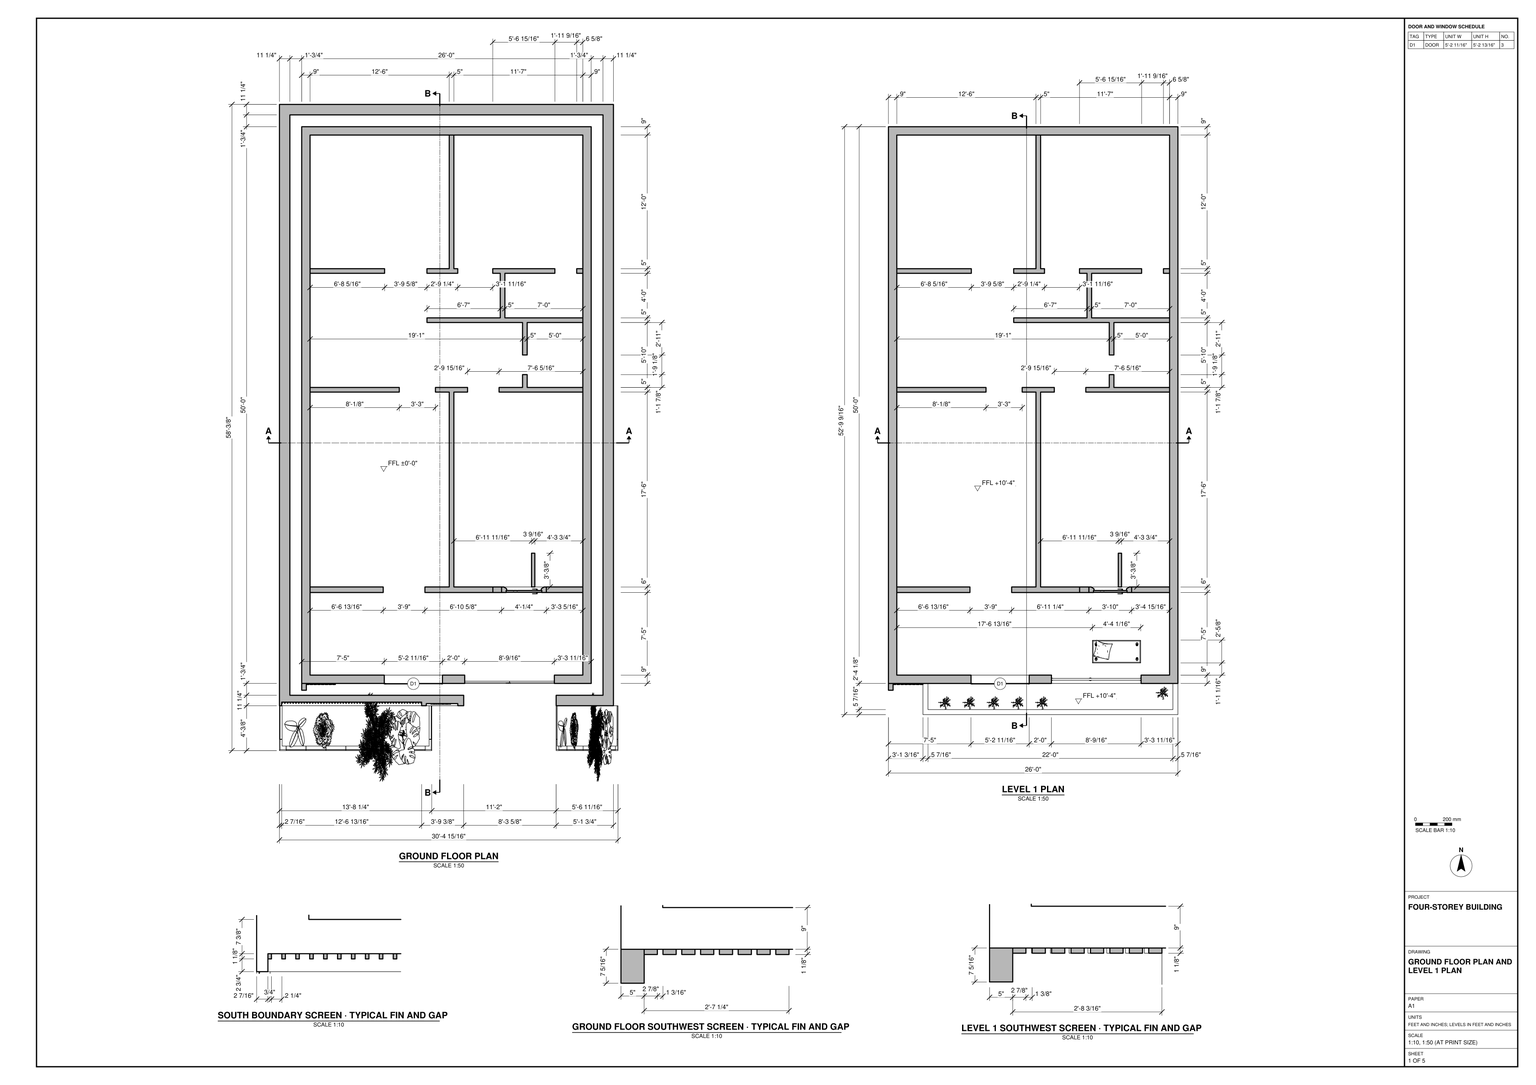
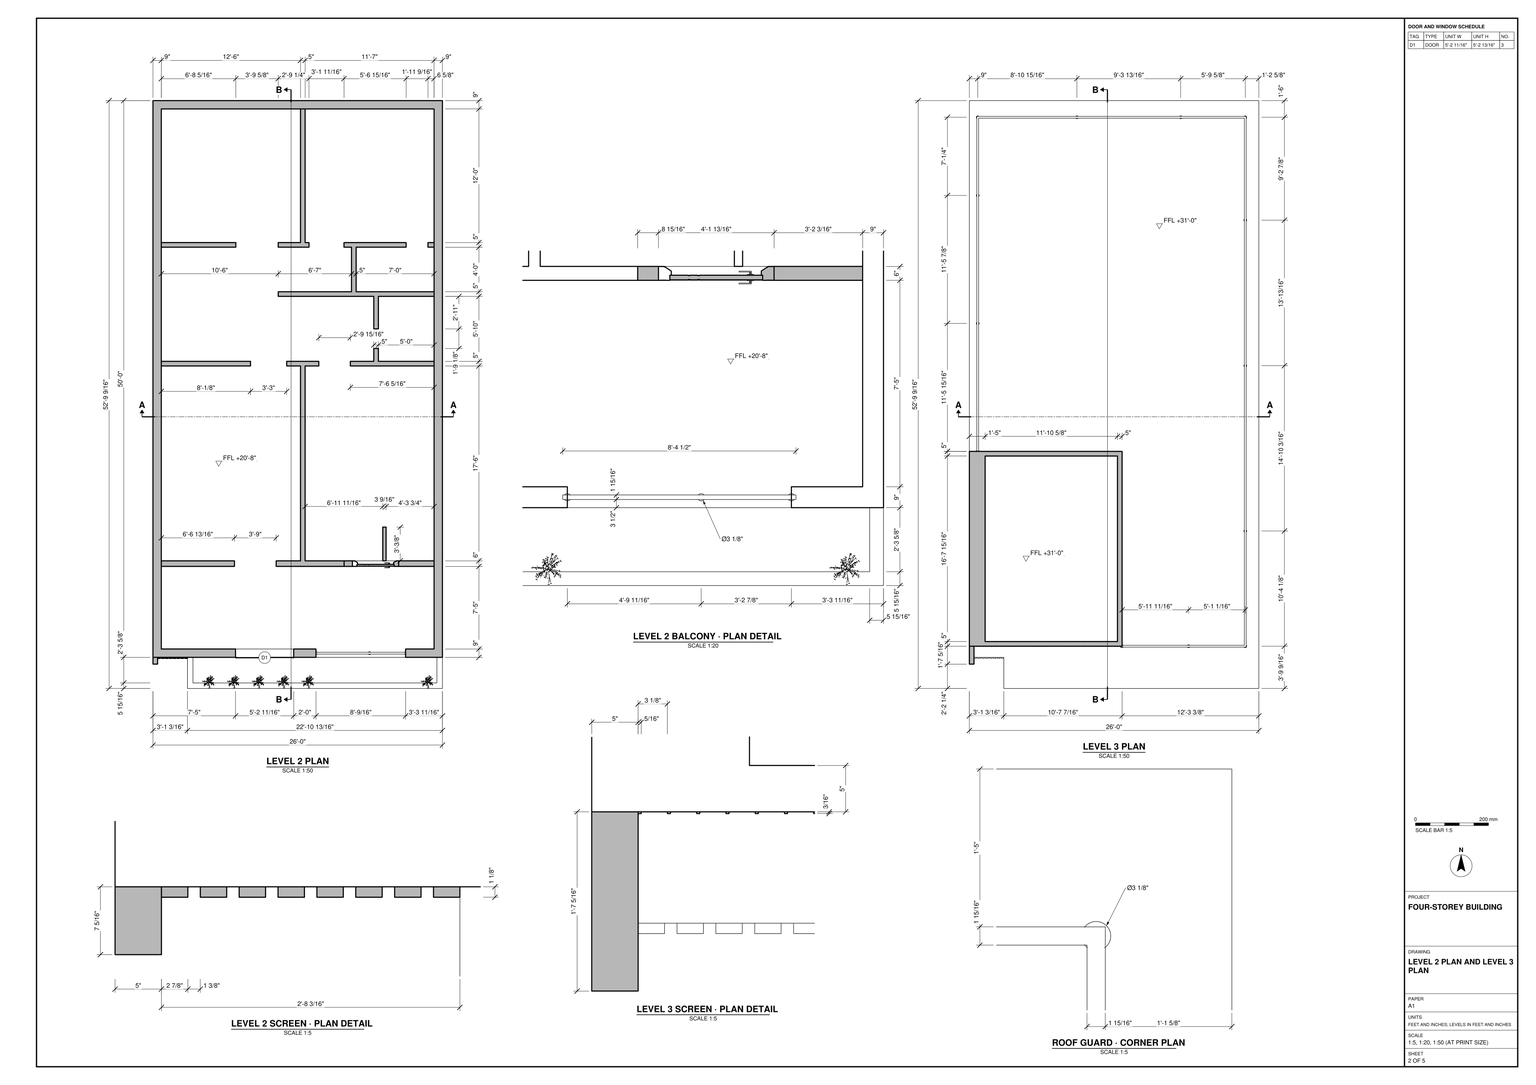
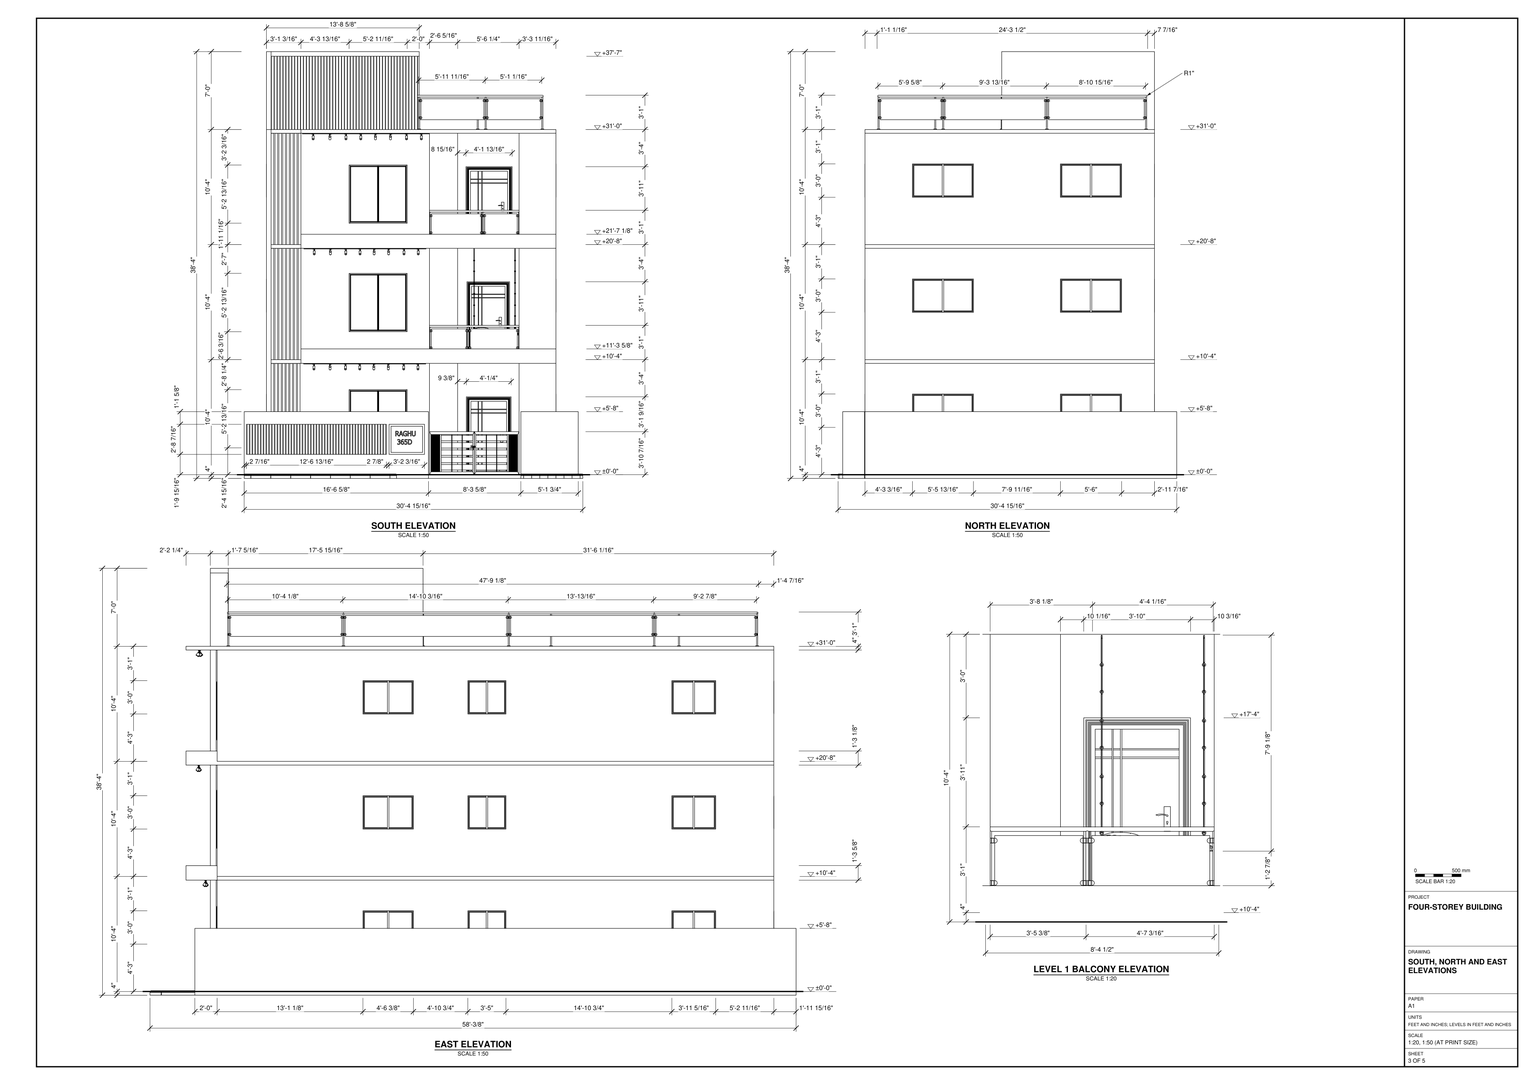
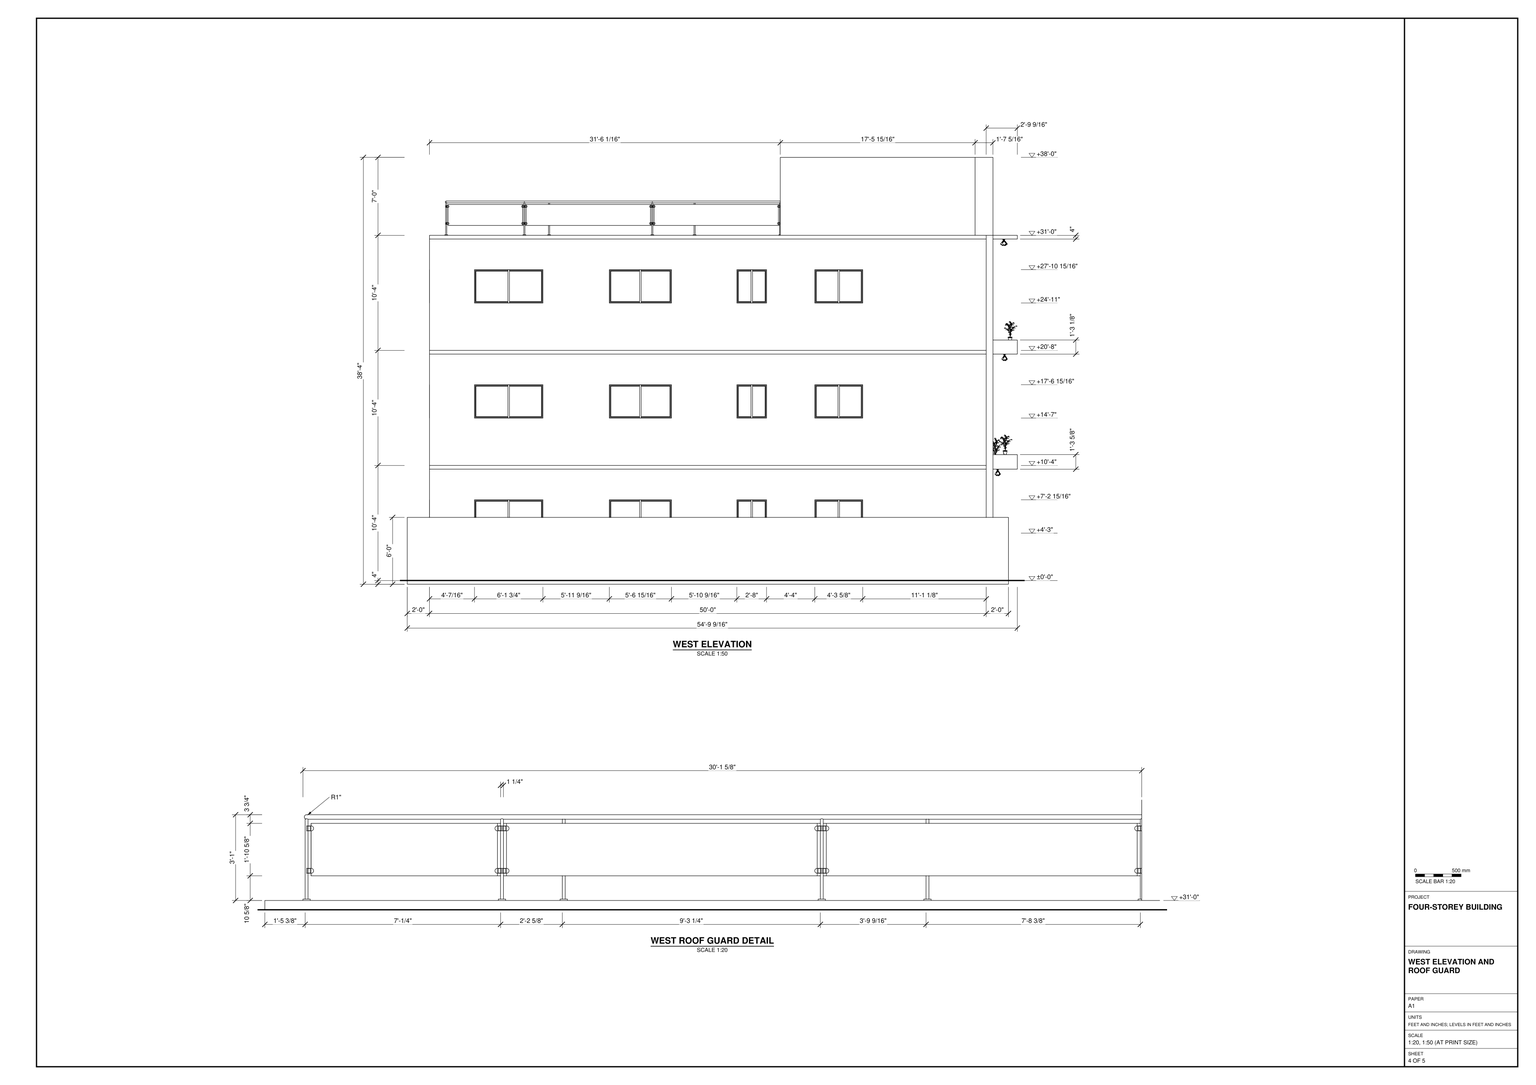
Build the four-storey building in SketchUp from task_files/diagram_01.pdf. Work in feet and inches, with the south entrance frontage along X and the building depth along Y. The overall model, including the boundary and frontage elements, is 30'-4 15/16" wide, 60'-9 5/8" deep and 38'-4" high. Set the finished floor levels to ±0'-0", +10'-4", +20'-8" and +31'-0".

Use the plans to set out the three lower floors. Model the perimeter walls, internal partitions and floor slabs at the thicknesses drawn. Preserve the passage openings between rooms, and use the elevations to place the exterior doors and windows. Model the projecting south balcony slabs, their guards and the narrow band of vertical fins at the southwest corner. At the top level, distinguish the screened southwest enclosure from the open roof terrace and follow the roof guard detail around the exposed edges.

Include the boundary walls, south entrance gate, finned boundary screen and planting beds in their plan positions. Place the swing shown near the southeast corner of the Level 1 front room. Model circulation, built-in joinery and main furniture where indicated on the sheets. Decor and loose items, including plants and lights, may be represented by any suitable library components.

Keep shell elements such as walls, slabs and roof separate as groups or components, and group each furniture or joinery piece separately. Use components for repeated parts such as screen fins and window units. Save one SketchUp model as output_files/four_storey_building_south_balconies_and_roof_terrace.skp.

# SketchUp Ruby script. Lengths in inches.
U = 1.inch
M = Sketchup.active_model
def pt(a) = Geom::Point3d.new(a.map { |v| v * U })
def face(e, loops, mat)
  f = e.add_face(loops[0].map { |a| pt(a) })
  loops[1..].each { |l| e.add_face(l.map { |a| pt(a) }).erase! }
  f.material = f.back_material = mat if mat
  f
end
# faces: each face lists its corners as indices into pts; further lists are holes
def faces(e, pts, list, mat = nil) = list.each { |f| face(e, (f[0].is_a?(Array) ? f : [f]).map { |l| l.map { |i| pts[i] } }, mat) }
# xy, xz, yz: faces in a plane at the given z, y or x. An outline is a flat list of corners, or four numbers for a rectangle; further outlines are holes
def ring(l) = l.size == 4 ? [[l[0], l[1]], [l[2], l[1]], [l[2], l[3]], [l[0], l[3]]] : l.each_slice(2).to_a
def flat(e, list, mat, &to3) = list.each { |f| face(e, (f[0].is_a?(Array) ? f : [f]).map { |l| ring(l).map { |u, v| to3.(u, v) } }, mat) }
def xy(e, z, list, mat = nil) = flat(e, list, mat) { |x, y| [x, y, z] }
def xz(e, y, list, mat = nil) = flat(e, list, mat) { |x, z| [x, y, z] }
def yz(e, x, list, mat = nil) = flat(e, list, mat) { |y, z| [x, y, z] }
def lines(e, pts, list) = list.each { |a, b| e.add_line(pt(pts[a]), pt(pts[b])) }
# prism: a flat outline (further loops are holes) pulled along v
def prism(e, loops, v, mat = nil)
  f = face(e, loops, mat); d = Geom::Vector3d.new(v.map { |x| x * U })
  f.pushpull(f.normal.samedirection?(d) ? d.length : -d.length)
end
def box(e, o, s, mat = nil) = prism(e, [[o, [o[0] + s[0], o[1], o[2]], [o[0] + s[0], o[1] + s[1], o[2]], [o[0], o[1] + s[1], o[2]]]], [0, 0, s[2]], mat)
def at(x, y, z, deg = 0) = Geom::Transformation.translation(pt([x, y, z])) * Geom::Transformation.rotation(ORIGIN, Z_AXIS, deg.degrees)
def axes(o, x, y, z) = Geom::Transformation.new([*x, 0, *y, 0, *z, 0, *pt(o).to_a, 1])
def part(name) = M.definitions.add(name)
# library, detail: a bought-in or finely detailed component or shape, given as its bounding box
def library(name, o, s) = part(name).tap { |d| box(d.entities, o, s) }
def detail(e, o, s) = box(e.add_group.entities, o, s)
def put(e, d, t, mat = nil) = e.add_instance(d, t).tap { |i| i.material = mat if mat }
def group(e, t, mat = nil) = e.add_group.tap { |g| g.transformation = t; g.material = mat if mat }.entities
root = M.entities
M.materials.add("PDM_Concrete_02N").color = [160, 160, 159]
M.materials.add("PDM_Concrete_02N-1").color = [160, 160, 159]
M.materials.add("PDM_Grass_03").color = [113, 137, 58]
M.materials.add("[0022_Maroon]").color = [128, 0, 0]
M.materials.add("[0041_Chocolate]").color = [210, 105, 30]
M.materials.add("[0132_LightGray]").color = [169, 169, 169]
M.materials.add("[0135_DarkGray]").color = [81, 81, 81]
M.materials.add("[0136_Charcoal]").color = [35, 35, 35]
M.materials.add("[Marble Carrara Floor Tile]").color = [204, 208, 219]
M.materials.add("[Mirror 02]").color = [229, 229, 229]
M.materials.add("[Terrazzo Light Blue]").color = [196, 214, 227]
M.materials.add("[Translucent Glass Tinted]").color = [8, 201, 241]
M.materials["[Translucent Glass Tinted]"].alpha = 0.48
M.materials.add("[Wood Cherry Original]").color = [152, 86, 42]
c1 = part("PENTEK_RP Fineline 50S_Sliding_DoorCase_E1")
box(c1.entities,[0,0,0],[1.51,3.66,99.27],"[0135_DarkGray]")
c2 = part("PENTEK_RP Fineline 50S_SlidingDooe_Case_E2")
box(c2.entities,[0,0,0],[96.25,3.66,1.51],"[0135_DarkGray]")
c3 = part("pentek_RP Fineline 50S_SlidingDoor_Case")
put(c3.entities,c1,at(97.76,0,0))
put(c3.entities,c2,at(1.51,0,0))
put(c3.entities,c1,at(0,0,0))
put(c3.entities,c2,at(1.51,0,97.76))
c4 = part("PENTEK_RP Fineline 50S_SlidingDoor_GlazingBead_2")
box(c4.entities,[0,0,0],[0.56,0.59,94.39],"[0135_DarkGray]")
c5 = part("PENTEK_RP Fineline 50S_SlidingDoor_Glass")
box(c5.entities,[0,0,0],[46.58,0.16,94.39],"[Translucent Glass Tinted]")
c6 = part("PENTEK_RP Fineline 50S_SlidingDoor_GlazingBead")
box(c6.entities,[0,0,0],[45.47,0.59,0.56],"[0135_DarkGray]")
c7 = part("PENTEK_RP Fineline 50S_SlidingDoor_Leaf_E1")
xy(c7.entities,0,[[0,0,0.93,1.97],[0.93,1.57,1.49,1.97]],"[0135_DarkGray]")
xy(c7.entities,96.25,[[0,0,0.93,0,0.93,1.57,1.49,1.57,1.49,1.97,0,1.97]],"[0135_DarkGray]")
xz(c7.entities,0,[[0,0,0.93,96.25]],"[0135_DarkGray]")
xz(c7.entities,1.57,[[0.93,0,1.49,95.32],[0.93,95.32,1.49,96.25]],"[0135_DarkGray]")
xz(c7.entities,1.97,[[0,0,1.49,96.25]],"[0135_DarkGray]")
yz(c7.entities,0,[[0,0,1.97,96.25]],"[0135_DarkGray]")
yz(c7.entities,0.93,[[0,0,1.57,0.93],[0,0.93,1.57,95.32],[0,95.32,1.57,96.25]],"[0135_DarkGray]")
yz(c7.entities,1.49,[[1.57,0,1.97,95.32],[1.57,95.32,1.97,96.25]],"[0135_DarkGray]")
c8 = part("PENTEK_RP Fineline 50S_SlidingDoor_Leaf_E2")
xy(c8.entities,0,[[0,0,0,1.57,0.56,1.57,0.56,1.97,46.02,1.97,46.02,1.57,46.58,1.57,46.58,0]],"[0135_DarkGray]")
xy(c8.entities,0.93,[[0,0,46.58,1.57]],"[0135_DarkGray]")
xy(c8.entities,1.49,[[0.56,1.57,46.02,1.97]],"[0135_DarkGray]")
xz(c8.entities,0,[[0,0,46.58,0.93]],"[0135_DarkGray]")
xz(c8.entities,1.57,[[0,0,0.56,0.93],[46.02,0,46.58,0.93],[0.56,0.93,46.02,1.49]],"[0135_DarkGray]")
xz(c8.entities,1.97,[[0.56,0,46.02,1.49]],"[0135_DarkGray]")
yz(c8.entities,0,[[0,0,1.57,0.93]],"[0135_DarkGray]")
yz(c8.entities,0.56,[[1.57,0,1.97,0.93],[1.57,0.93,1.97,1.49]],"[0135_DarkGray]")
yz(c8.entities,46.02,[[1.57,0,1.97,0.93],[1.57,0.93,1.97,1.49]],"[0135_DarkGray]")
yz(c8.entities,46.58,[[0,0,1.57,0.93]],"[0135_DarkGray]")
c9 = part("PENTEK_RP Fineline S_SlidingDoor_Leaf1")
put(c9.entities,c4,at(0.93,0,0.93))
put(c9.entities,c4,at(46.96,0,0.93))
put(c9.entities,c5,at(1.49,1.42,0.93))
put(c9.entities,c6,at(1.49,0,0.93))
put(c9.entities,c5,at(1.49,0.59,0.93),"[Terrazzo Light Blue]")
put(c9.entities,c7,at(0,0,0))
put(c9.entities,c7,axes([48.44,0,0],[-1,0,0],[0,1,0],[0,0,1]))
put(c9.entities,c8,axes([0.93,0,96.25],[1,0,0],[0,1,0],[0,0,-1]))
put(c9.entities,c8,at(0.93,0,0))
put(c9.entities,c6,at(1.49,0,94.77))
c10 = part("PENTEK_RP Fineline 50S_SlidingDoor_Leaf2")
put(c10.entities,c5,at(1.49,1.42,0.93))
put(c10.entities,c6,at(1.49,0,94.77))
put(c10.entities,c4,at(46.96,0,0.93))
put(c10.entities,c5,at(1.49,0.59,0.93),"[Mirror 02]")
put(c10.entities,c4,at(0.93,0,0.93))
put(c10.entities,c7,at(0,0,0))
put(c10.entities,c7,axes([48.44,0,0],[-1,0,0],[0,1,0],[0,0,1]))
put(c10.entities,c6,at(1.49,0,0.93))
put(c10.entities,c8,axes([0.93,0,96.25],[1,0,0],[0,1,0],[0,0,-1]))
put(c10.entities,c8,at(0.93,0,0))
c11 = part("PENTEK - Slimmest Steel Sliding Door / Window\#1")
put(c11.entities,c3,at(0,-1.88,-0.09))
put(c11.entities,c9,at(1.51,-2.27,1.42),"[0041_Chocolate]")
put(c11.entities,c10,at(49.32,-0.3,1.42),"[0041_Chocolate]")
c12 = library("track spot lights",[-0.02,-0.08,0],[184.83,7.92,7.16])
c13 = part("Group136\#1")
p = [[0,0,0],[0,0,-16.31],[-4.35,0,-16.31],[28.32,-24.48,0],[-28.32,-24.48,0],[28.32,24.48,0],
  [28.32,0,0],[-28.32,24.48,0],[4.35,0,-16.31],[-28.32,0,0],[0,0,-26.4]]
lines(c13.entities,p,[[0,1],[1,2],[3,4],[5,6],[7,5],[1,8],[9,0],[0,6],[8,10],[4,9],[6,3],[2,10],
  [9,7]])
c14 = part("Rectangle Light")
put(c14.entities,c13,at(0,0,0))
c15 = part("Group138\#1")
p = [[0,0,0],[0,0,-9.13],[-1.42,0,-9.13],[9.23,-20.33,0],[-9.23,-20.33,0],[9.23,20.33,0],
  [9.23,0,0],[-9.23,20.33,0],[1.42,0,-9.13],[-9.23,0,0],[0,0,-14.78]]
lines(c15.entities,p,[[0,1],[1,2],[3,4],[5,6],[7,5],[1,8],[9,0],[0,6],[8,10],[4,9],[6,3],[2,10],
  [9,7]])
c16 = part("Rectangle Light\#1")
put(c16.entities,c15,at(0,0,0))
c17 = part("Group140\#1")
p = [[0,0,0],[0,0,-16.18],[-6.125,0,-16.18],[39.875,-12.51,0],[-39.875,-12.51,0],[39.875,12.51,0],
  [39.875,0,0],[-39.875,12.51,0],[6.125,0,-16.18],[-39.875,0,0],[0,0,-26.19]]
lines(c17.entities,p,[[0,1],[1,2],[3,4],[5,6],[7,5],[1,8],[9,0],[0,6],[8,10],[4,9],[6,3],[2,10],
  [9,7]])
c18 = part("Rectangle Light\#2")
put(c18.entities,c17,at(0,0,0))
c19 = part("Group142\#1")
p = [[0,0,0],[0,0,-9.18],[-1.75,0,-9.18],[11.4,-18.32,0],[-11.4,-18.32,0],[11.4,18.32,0],
  [11.4,0,0],[-11.4,18.32,0],[1.75,0,-9.18],[-11.4,0,0],[0,0,-14.86]]
lines(c19.entities,p,[[0,1],[1,2],[3,4],[5,6],[7,5],[1,8],[9,0],[0,6],[8,10],[4,9],[6,3],[2,10],
  [9,7]])
c20 = part("Rectangle Light\#3")
put(c20.entities,c19,at(0,0,0))
c21 = part("Group144\#1")
p = [[0,0,0],[0,0,-17.3125],[-6.92,0,-17.3125],[45.07,-10.98,0],[-45.07,-10.98,0],[45.07,10.98,0],
  [45.07,0,0],[-45.07,10.98,0],[6.92,0,-17.3125],[-45.07,0,0],[0,0,-28.02]]
lines(c21.entities,p,[[0,1],[1,2],[3,4],[5,6],[7,5],[1,8],[9,0],[0,6],[8,10],[4,9],[6,3],[2,10],
  [9,7]])
c22 = part("Rectangle Light\#4")
put(c22.entities,c21,at(0,0,0))
c23 = part("Group146\#1")
p = [[0,0,0],[0,0,-17.125],[-5.35,0,-17.125],[34.8,-20.64,0],[-34.8,-20.64,0],[34.8,20.64,0],
  [34.8,0,0],[-34.8,20.64,0],[5.35,0,-17.125],[-34.8,0,0],[0,0,-27.72]]
lines(c23.entities,p,[[0,1],[1,2],[3,4],[5,6],[7,5],[1,8],[9,0],[0,6],[8,10],[4,9],[6,3],[2,10],
  [9,7]])
c24 = part("Rectangle Light\#5")
put(c24.entities,c23,at(0,0,0))
c25 = part("255x125 HB kerb.skp\#1")
prism(c25.entities,[[[35.98,4.92,10.04],[35.98,1.15,10.04],[35.98,0.9375,9.96],[35.98,0.8125,9.77],[35.98,0,6.1],[35.98,0,0],[35.98,4.92,0]]],[-35.98,0,0])
c26 = part("305x125 HB external kerb.skp")
xy(c26.entities,0,[[0,0,0,4.92,7.09,4.92,7.09,12.01,12.01,12.01,12.01,0]])
xy(c26.entities,10.04,[[0,1.15,10.86,1.15,10.86,12.01,7.09,12.01,7.09,4.92,0,4.92]])
xz(c26.entities,0,[[0,0,12.01,6.1]])
xz(c26.entities,4.92,[[0,0,7.09,10.04]])
xz(c26.entities,12.01,[[7.09,0,7.09,10.04,10.86,10.04,11.07,9.96,11.19,9.77,12.01,6.1,12.01,0]])
yz(c26.entities,0,[[0,0,0,6.1,0.8125,9.77,0.9375,9.96,1.15,10.04,4.92,10.04,4.92,0]])
yz(c26.entities,7.09,[[4.92,0,12.01,10.04]])
yz(c26.entities,12.01,[[0,0,12.01,6.1]])
p = [[0,0.8125,9.77],[0,0,6.1],[12.01,0,6.1],[11.19,0.8125,9.77],[12.01,12.01,6.1],[11.19,12.01,9.77],
  [0,0.9375,9.96],[11.07,0.9375,9.96],[11.07,12.01,9.96],[0,1.15,10.04],[10.86,1.15,10.04],[10.86,12.01,10.04]]
faces(c26.entities,p,[[0,1,2,3],[3,2,4,5],[6,0,3,7],[7,3,5,8],[9,6,7,10],[10,7,8,11]])
c27 = library("Vase_plant.skp",[-29.68,-24.2,-1.65],[45.82,40.28,40.94])
c28 = library("Aralia.skp\#1",[-13.5,-14.26,0],[27.8,28.98,28.64])
c29 = library("bamboo2.skp\#1",[-10.58,-11.09,0],[94.17,118.22,79.29])
c30 = library("Monstera.skp\#1",[-40.08,-33.23,-2.65],[72.39,71.54,61.35])
c31 = part("flowers")
xy(c31.entities,8.27,[[6.7,5.98,275.44,49.6875]],"PDM_Grass_03")
xz(c31.entities,5.98,[[6.7,0,275.44,8.27]])
xz(c31.entities,49.6875,[[6.7,0,6.9375,8.27],[6.9375,0,275.44,8.27],[6.9375,8.27,275.44,10.04]],"PDM_Concrete_02N")
yz(c31.entities,6.7,[[5.98,0,49.6875,8.27]])
yz(c31.entities,275.44,[[5.98,0,49.6875,8.27]])
p = [[2.02,1.3,0],[2.02,40.67,0]]
lines(c31.entities,p,[[0,1]])
put(c31.entities,c25,at(14.42,1.3,0),"PDM_Concrete_02N-1")
put(c31.entities,c26,at(268.36,1.3,0),"PDM_Concrete_02N-1")
put(c31.entities,c26,at(2.02,13.31,0,-90),"PDM_Concrete_02N-1")
put(c31.entities,c25,at(50.8,1.3,0),"PDM_Concrete_02N-1")
put(c31.entities,c25,at(87.18,1.3,0),"PDM_Concrete_02N-1")
put(c31.entities,c25,at(123.55,1.3,0),"PDM_Concrete_02N-1")
put(c31.entities,c25,at(159.77,1.3,0),"PDM_Concrete_02N-1")
put(c31.entities,c25,at(195.99,1.3,0),"PDM_Concrete_02N-1")
put(c31.entities,c25,at(232.21,1.3,0),"PDM_Concrete_02N-1")
put(c31.entities,c25,at(280.36,13.7,0,90),"PDM_Concrete_02N-1")
put(c31.entities,c25,at(2.02,49.6875,0,-90),"PDM_Concrete_02N-1")
put(c31.entities,c27,at(36.73,27.57,8.27))
put(c31.entities,c28,axes([82.45,23.77,8.27],[1.4,0,0],[0,1.43,0],[0,0,1.63]))
put(c31.entities,c29,at(140.88,-31.91,8.22))
put(c31.entities,c30,at(227.05,18.7,8.27,-180))
c32 = library("TRADITIONAL SWING",[0,0,0],[52.04,24.99,103.38])
c33 = part("Group\#6")
box(c33.entities,[0,0,0],[6.61,5,120])
c34 = part("Group\#9")
box(c34.entities,[0,0,0],[3.5625,36.37,120])
c35 = part("Group\#7")
prism(c35.entities,[[[33.23,5,0],[33.23,0,0],[0,0,0],[0,5,0],[24.03,5,0],[24.03,149,0],[29.03,149,0],[29.03,5,0]]],[0,0,120])
c36 = part("Group\#8")
box(c36.entities,[0,0,0],[96.15,5,120])
c37 = library("Group\#42",[0,-1.57,0],[96.98,7.57,120])
c38 = part("Group\#3")
prism(c38.entities,[[[0,40,0],[79,40,0],[79,88,0],[70.89,88,0],[70.89,93,0],[137.86,93,0],[137.86,88,0],[84,88,0],[84,40,0],[168,40,0],[168,35,0],[108,35,0],[108,0,0],[103,0,0],[103,35,0],[0,35,0]]],[0,0,120])
c39 = part("Group\#4")
box(c39.entities,[0,0,0],[80.33,5,120])
c40 = part("Group\#5")
prism(c40.entities,[[[25.29,18.85,0],[30.29,18.85,0],[30.29,5,0],[90.29,5,0],[90.29,0,0],[0,0,0],[0,5,0],[25.29,5,0]]],[0,0,120])
c41 = part("Group\#10")
prism(c41.entities,[[[78.84,6,0],[78.84,0,0],[0,0,0],[0,6,0],[36.22,6,0]]],[0,0,120])
c42 = library("Group\#14",[0,0,0],[9.07,41.0625,36])
c43 = library("Group\#28",[0,0,0],[9.07,51.68,36])
c44 = part("Difference\#4")
xy(c44.entities,0,[[0,0,0,600,312,600,312,0,272.29,0,272.29,9,303,9,303,591,9,591,9,9,175.7,9,175.7,0]])
xy(c44.entities,30.1875,[[89,0,151.7,9]])
xy(c44.entities,51,[[0,133.0625,9,184.74],[303,157.16,312,211.54],[0,236.68,9,268.72],[303,270.25,312,311.31],[0,339.22,9,406.21],
  [0,477.75,9,551.55],[303,490.05,312,537.4],[35.41,591,101.4,600],[195.08,591,260.875,600]])
xy(c44.entities,87,[[0,133.0625,9,184.74],[303,157.16,312,211.54],[0,236.68,9,268.72],[303,270.25,312,311.31],[0,339.22,9,406.21],
  [0,477.75,9,551.55],[303,490.05,312,537.4],[35.41,591,101.4,600],[195.08,591,260.875,600]])
xy(c44.entities,92.89,[[89,0,151.7,9]])
xy(c44.entities,120,[[0,0,175.7,0,175.7,9,9,9,9,591,303,591,303,9,272.29,9,272.29,0,312,0,312,600,0,600]])
xz(c44.entities,0,[[[0,0,175.7,120],[89,30.1875,151.7,92.89]],[272.29,0,312,120]])
xz(c44.entities,9,[[[9,0,175.7,120],[89,30.1875,151.7,92.89]],[272.29,0,303,120]])
xz(c44.entities,133.0625,[[0,51,9,87]])
xz(c44.entities,157.16,[[303,51,312,87]])
xz(c44.entities,184.74,[[0,51,9,87]])
xz(c44.entities,211.54,[[303,51,312,87]])
xz(c44.entities,236.68,[[0,51,9,87]])
xz(c44.entities,268.72,[[0,51,9,87]])
xz(c44.entities,270.25,[[303,51,312,87]])
xz(c44.entities,311.31,[[303,51,312,87]])
xz(c44.entities,339.22,[[0,51,9,87]])
xz(c44.entities,406.21,[[0,51,9,87]])
xz(c44.entities,477.75,[[0,51,9,87]])
xz(c44.entities,490.05,[[303,51,312,87]])
xz(c44.entities,537.4,[[303,51,312,87]])
xz(c44.entities,551.55,[[0,51,9,87]])
xz(c44.entities,591,[[[9,0,303,120],[35.41,51,101.4,87],[195.08,51,260.875,87]]])
xz(c44.entities,600,[[[0,0,312,120],[35.41,51,101.4,87],[195.08,51,260.875,87]]])
yz(c44.entities,0,[[[0,0,600,120],[477.75,51,551.55,87],[339.22,51,406.21,87],[133.0625,51,184.74,87],[236.68,51,268.72,87]]])
yz(c44.entities,9,[[[9,0,591,120],[477.75,51,551.55,87],[339.22,51,406.21,87],[133.0625,51,184.74,87],[236.68,51,268.72,87]]])
yz(c44.entities,35.41,[[591,51,600,87]])
yz(c44.entities,89,[[0,30.1875,9,92.89]])
yz(c44.entities,101.4,[[591,51,600,87]])
yz(c44.entities,151.7,[[0,30.1875,9,92.89]])
yz(c44.entities,175.7,[[0,0,9,120]])
yz(c44.entities,195.08,[[591,51,600,87]])
yz(c44.entities,260.875,[[591,51,600,87]])
yz(c44.entities,272.29,[[0,0,9,120]])
yz(c44.entities,303,[[[9,0,591,120],[157.16,51,211.54,87],[490.05,51,537.4,87],[270.25,51,311.31,87]]])
yz(c44.entities,312,[[[0,0,600,120],[157.16,51,211.54,87],[490.05,51,537.4,87],[270.25,51,311.31,87]]])
c45 = library("Group\#24",[0,0,0],[9.07,66.99,36])
c46 = library("Group\#26",[0,0,0],[9.07,32.04,36])
c47 = library("Group\#12",[0,0,0],[9.07,54.39,36])
c48 = library("Group\#16",[0,0,0],[9.07,47.35,36])
c49 = library("Group\#22",[0,0,0],[9.07,73.8,36])
c50 = library("Group\#18",[0,0,0],[65.79,9.07,36])
c51 = library("Group\#20",[0,0,0],[65.99,9.07,36])
c52 = library("Group\#61",[-0.5,-0.5,0],[67.8125,105.9375,1.1875])
c53 = library("Group\#44",[0,-1.57,0],[96.98,7.57,120])
c54 = part("Difference")
xy(c54.entities,0,[[0,0,0,600,312,600,312,0,272.29,0,272.29,9,303,9,303,591,9,591,9,9,175.7,9,175.7,0]])
xy(c54.entities,24,[[89,0,151.7,9]])
xy(c54.entities,51,[[0,133.0625,9,184.74],[303,157.16,312,211.54],[0,236.68,9,268.72],[303,270.25,312,311.31],[0,339.22,9,406.21],
  [0,477.75,9,551.55],[303,490.05,312,537.4],[35.41,591,101.4,600],[195.08,591,260.875,600]])
xy(c54.entities,84,[[89,0,151.7,9]])
xy(c54.entities,87,[[0,133.0625,9,184.74],[303,157.16,312,211.54],[0,236.68,9,268.72],[303,270.25,312,311.31],[0,339.22,9,406.21],
  [0,477.75,9,551.55],[303,490.05,312,537.4],[35.41,591,101.4,600],[195.08,591,260.875,600]])
xy(c54.entities,120,[[0,0,175.7,0,175.7,9,9,9,9,591,303,591,303,9,272.29,9,272.29,0,312,0,312,600,0,600]])
xz(c54.entities,0,[[[0,0,175.7,120],[89,24,151.7,84]],[272.29,0,312,120]])
xz(c54.entities,9,[[[9,0,175.7,120],[89,24,151.7,84]],[272.29,0,303,120]])
xz(c54.entities,133.0625,[[0,51,9,87]])
xz(c54.entities,157.16,[[303,51,312,87]])
xz(c54.entities,184.74,[[0,51,9,87]])
xz(c54.entities,211.54,[[303,51,312,87]])
xz(c54.entities,236.68,[[0,51,9,87]])
xz(c54.entities,268.72,[[0,51,9,87]])
xz(c54.entities,270.25,[[303,51,312,87]])
xz(c54.entities,311.31,[[303,51,312,87]])
xz(c54.entities,339.22,[[0,51,9,87]])
xz(c54.entities,406.21,[[0,51,9,87]])
xz(c54.entities,477.75,[[0,51,9,87]])
xz(c54.entities,490.05,[[303,51,312,87]])
xz(c54.entities,537.4,[[303,51,312,87]])
xz(c54.entities,551.55,[[0,51,9,87]])
xz(c54.entities,591,[[[9,0,303,120],[35.41,51,101.4,87],[195.08,51,260.875,87]]])
xz(c54.entities,600,[[[0,0,312,120],[35.41,51,101.4,87],[195.08,51,260.875,87]]])
yz(c54.entities,0,[[[0,0,600,120],[477.75,51,551.55,87],[339.22,51,406.21,87],[133.0625,51,184.74,87],[236.68,51,268.72,87]]])
yz(c54.entities,9,[[[9,0,591,120],[477.75,51,551.55,87],[339.22,51,406.21,87],[133.0625,51,184.74,87],[236.68,51,268.72,87]]])
yz(c54.entities,35.41,[[591,51,600,87]])
yz(c54.entities,89,[[0,24,9,84]])
yz(c54.entities,101.4,[[591,51,600,87]])
yz(c54.entities,151.7,[[0,24,9,84]])
yz(c54.entities,175.7,[[0,0,9,120]])
yz(c54.entities,195.08,[[591,51,600,87]])
yz(c54.entities,260.875,[[591,51,600,87]])
yz(c54.entities,272.29,[[0,0,9,120]])
yz(c54.entities,303,[[[9,0,591,120],[157.16,51,211.54,87],[490.05,51,537.4,87],[270.25,51,311.31,87]]])
yz(c54.entities,312,[[[0,0,600,120],[157.16,51,211.54,87],[490.05,51,537.4,87],[270.25,51,311.31,87]]])
c55 = library("Group\#59",[-0.5,-0.5,0],[71.75,93.1875,2.8125])
c56 = library("RAGHU  365D",[0.29,0,0],[12.08,7.7,1])
c57 = library("Group\#50",[0,0,0],[100.53,3.15,36.98])
c58 = library("Group\#49",[0,0,0],[100.53,3.15,36.98])
c59 = library("Group\#51",[0,0,0],[291.52,573.15,36.98])
c60 = library("Group\#52",[0,0,0],[164.63,19.3125,456])
c61 = part("Group\#53")
box(c61.entities,[0,0,0],[0.33,0.1875,79])
c62 = part("Difference\#5")
xy(c62.entities,0,[[0,0,0,600,312,600,312,0,272.29,0,272.29,9,303,9,303,591,9,591,9,9,175.7,9,175.7,0]])
xy(c62.entities,29.04,[[89,0,151.7,9]])
xy(c62.entities,51,[[0,133.0625,9,184.74],[303,157.16,312,211.54],[0,236.68,9,268.72],[303,270.25,312,311.31],[0,339.22,9,406.21],
  [0,477.75,9,551.55],[303,490.05,312,537.4],[35.41,591,101.4,600],[195.08,591,260.875,600]])
xy(c62.entities,87,[[0,133.0625,9,184.74],[303,157.16,312,211.54],[0,236.68,9,268.72],[303,270.25,312,311.31],[0,339.22,9,406.21],
  [0,477.75,9,551.55],[303,490.05,312,537.4],[35.41,591,101.4,600],[195.08,591,260.875,600]])
xy(c62.entities,91.74,[[89,0,151.7,9]])
xy(c62.entities,120,[[0,0,175.7,0,175.7,9,9,9,9,591,303,591,303,9,272.29,9,272.29,0,312,0,312,600,0,600]])
xz(c62.entities,0,[[[0,0,175.7,120],[89,29.04,151.7,91.74]],[272.29,0,312,120]])
xz(c62.entities,9,[[[9,0,175.7,120],[89,29.04,151.7,91.74]],[272.29,0,303,120]])
xz(c62.entities,133.0625,[[0,51,9,87]])
xz(c62.entities,157.16,[[303,51,312,87]])
xz(c62.entities,184.74,[[0,51,9,87]])
xz(c62.entities,211.54,[[303,51,312,87]])
xz(c62.entities,236.68,[[0,51,9,87]])
xz(c62.entities,268.72,[[0,51,9,87]])
xz(c62.entities,270.25,[[303,51,312,87]])
xz(c62.entities,311.31,[[303,51,312,87]])
xz(c62.entities,339.22,[[0,51,9,87]])
xz(c62.entities,406.21,[[0,51,9,87]])
xz(c62.entities,477.75,[[0,51,9,87]])
xz(c62.entities,490.05,[[303,51,312,87]])
xz(c62.entities,537.4,[[303,51,312,87]])
xz(c62.entities,551.55,[[0,51,9,87]])
xz(c62.entities,591,[[[9,0,303,120],[35.41,51,101.4,87],[195.08,51,260.875,87]]])
xz(c62.entities,600,[[[0,0,312,120],[35.41,51,101.4,87],[195.08,51,260.875,87]]])
yz(c62.entities,0,[[[0,0,600,120],[477.75,51,551.55,87],[339.22,51,406.21,87],[133.0625,51,184.74,87],[236.68,51,268.72,87]]])
yz(c62.entities,9,[[[9,0,591,120],[477.75,51,551.55,87],[339.22,51,406.21,87],[133.0625,51,184.74,87],[236.68,51,268.72,87]]])
yz(c62.entities,35.41,[[591,51,600,87]])
yz(c62.entities,89,[[0,29.04,9,91.74]])
yz(c62.entities,101.4,[[591,51,600,87]])
yz(c62.entities,151.7,[[0,29.04,9,91.74]])
yz(c62.entities,175.7,[[0,0,9,120]])
yz(c62.entities,195.08,[[591,51,600,87]])
yz(c62.entities,260.875,[[591,51,600,87]])
yz(c62.entities,272.29,[[0,0,9,120]])
yz(c62.entities,303,[[[9,0,591,120],[157.16,51,211.54,87],[490.05,51,537.4,87],[270.25,51,311.31,87]]])
yz(c62.entities,312,[[[0,0,600,120],[157.16,51,211.54,87],[490.05,51,537.4,87],[270.25,51,311.31,87]]])
c63 = library("Group\#1",[0,-1.57,0],[96.98,7.57,120])
c64 = library("Group\#62",[-0.5,-0.5,0],[62.3125,103.5625,2.875])
c65 = part("Group\#60")
box(c65.entities,[0,0,0],[2.84,1.125,119.89])
c66 = library("Group\#77",[-0.05,-0.05,0],[13.65,14.49,22.0625])
c67 = part("Group\#78")
box(c67.entities,[0,0,0],[0.77,1.125,32.4375])
c68 = library("Group\#98",[0,0,0],[2.41,197.24,46.46])
xy(root,244,[[222,51.83,224.95,156.76],[224.95,51.83,288.81,54.79],[285.81,54.83,288.81,156.76],[224.95,153.76,285.81,156.76]],"[Translucent Glass Tinted]")
p = [[336,672.39,-4],[24,672.39,-4],[24,72.39,-4],[336.46,72.39,-4],[336,72.39,124],[336,72.39,120]]
lines(root,p,[[0,1],[2,3],[2,1],[4,5]])
put(root,c11,axes([113,72.16,29.01],[0.63156,0,0],[0,0.12784,0],[0,0,0.63248]))
put(root,c11,axes([113,72.16,154.25],[0.63156,0,0],[0,0.12784,0],[0,0,0.63248]))
put(root,c11,axes([113,72.16,271.1],[0.63156,0,0],[0,0.12784,0],[0,0,0.63248]))
put(root,c12,axes([62.68,49.5,360.84],[0.74143,0,0],[0,1,0],[0,0,1]))
put(root,c12,axes([64.3,49.48,236.84],[0.7128,0,0],[0,0.81,0],[0,0,1]))
put(root,c12,axes([63.98,56.9,112.84],[0.7128,0,0],[0,0.81,0],[0,0,1]))
put(root,c14,axes([144.44,131.51,367.99],[-1,0,0],[0,1,0],[0,0,1]))
put(root,c16,at(99.7,255.39,367.99))
put(root,c18,axes([166.07,97.48,243.99],[1,0,0],[0,-1,0],[0,0,1]))
put(root,c20,at(120.12,222.72,243.99))
put(root,c22,axes([150.18,97.93,119.99],[1,0,0],[0,-1,0],[0,0,1]))
put(root,c24,axes([145.55,165.81,119.99],[1,0,0],[0,-1,0],[0,0,1]))
put(root,c31,axes([-1.19,-1.3,-4],[0.59,0,0],[0,1,0],[0,0,0.48152]))
put(root,c31,axes([297.74,-1.3,-4],[0.23968,0,0],[0,1,0],[0,0,0.48152]))
put(root,c32,axes([243.84,94.47,150.5],[1,0,0],[0,0.99741,0],[0,0,0.902]))
g1 = group(root,at(24,72.39,-4))
xy(g1,0,[[0,0,312,600]])
xy(g1,4,[[0,0,312,600]],"[Marble Carrara Floor Tile]")
xz(g1,0,[[0,0,312,4]])
xz(g1,600,[[0,0,312,4]])
yz(g1,0,[[0,0,600,4]])
yz(g1,312,[[0,0,600,4]])
g2 = group(root,at(23.93,72.39,124))
put(g2,c33,at(296.46,442,0))
g3 = group(g2,at(0,0,0))
g4 = group(g3,at(0,0,0))
put(g4,c34,at(247.77,104,0))
put(g4,c35,at(135.04,442,0))
put(g4,c36,at(9.07,314,0))
put(g4,c37,at(206.1,98,0))
g5 = group(g4,at(132.875,98,0))
prism(g5,[[[73.22,6,0],[73.22,0,0],[0,0,0],[0,6,0],[26.2,6,0],[26.2,216,0],[11.33,216,0],[11.33,221,0],[45.95,221,0],[45.95,216,0],[31.2,216,0],[31.2,6,0]]],[0,0,120])
put(g4,c38,at(135.07,354,0))
put(g4,c39,at(9.07,442,0))
put(g4,c40,at(212.78,314,0))
put(g4,c41,at(9.07,98,0))
g6 = group(g4,at(0,0,0))
put(g6,c42,at(312.14,311.31,51,180))
put(g6,c43,at(9.07,184.74,51,180))
put(g6,c44,at(0.07,0,0))
put(g6,c45,at(9.07,406.21,51,180))
put(g6,c46,at(9.07,268.72,51,180))
put(g6,c47,at(312.14,211.54,51,180))
put(g6,c48,at(312.14,537.4,51,180))
put(g6,c49,at(9.07,551.55,51,180))
put(g3,c50,at(260.95,600.07,51,180))
put(g3,c51,at(101.47,600.07,51,180))
g7 = group(root,at(24,72.39,244),"[0135_DarkGray]")
xy(g7,0,[[[37.17,-33.5625,37.17,0,0,0,0,600,312,600,312,-33.5625],[198,-20.56,264.81,84.38]],[201,-17.56,261.81,81.38]],"[Wood Cherry Original]")
xy(g7,4,[[43.12,-27.61,306.05,0]])
xy(g7,4,[[0,0,312,600]],"[Marble Carrara Floor Tile]")
xy(g7,15.125,[[37.17,-33.5625,312,-33.5625,312,0,306.05,0,306.05,-27.61,43.12,-27.61,43.12,0,37.17,0]])
xz(g7,-33.5625,[[37.17,0,312,15.125]])
xz(g7,-27.61,[[43.12,4,306.05,15.125]])
xz(g7,-20.56,[[198,0,264.81,1.1875]],"[Wood Cherry Original]")
xz(g7,0,[[0,0,37.17,4],[37.17,4,43.12,15.125],[306.05,4,312,15.125]])
xz(g7,81.38,[[201,0,261.81,1.1875]],"[Wood Cherry Original]")
xz(g7,600,[[0,0,312,4]])
yz(g7,0,[[0,0,600,4]])
yz(g7,37.17,[[-33.5625,0,0,15.125]])
yz(g7,43.12,[[-27.61,4,0,15.125]])
yz(g7,201,[[-17.56,0,81.38,1.1875]],"[Wood Cherry Original]")
yz(g7,306.05,[[-27.61,4,0,15.125]])
yz(g7,312,[[-33.5625,0,600,0,600,4,0,4,0,15.125,-33.5625,15.125]])
put(g7,c52,at(198,-20.56,0))
g8 = group(root,at(23.93,72.39,248))
put(g8,c33,at(296.46,442,0))
g9 = group(g8,at(0,0,0))
g10 = group(g9,at(0,0,0))
put(g10,c34,at(247.77,104,0))
put(g10,c35,at(135.04,442,0))
put(g10,c36,at(9.07,314,0))
put(g10,c53,at(206.1,98,0))
g11 = group(g10,at(132.875,98,0))
prism(g11,[[[73.22,6,0],[73.22,0,0],[0,0,0],[0,6,0],[26.2,6,0],[26.2,216,0],[11.33,216,0],[11.33,221,0],[45.95,221,0],[45.95,216,0],[31.2,216,0],[31.2,6,0]]],[0,0,120])
put(g10,c38,at(135.07,354,0))
put(g10,c39,at(9.07,442,0))
put(g10,c40,at(212.78,314,0))
put(g10,c41,at(9.07,98,0))
g12 = group(g10,at(0,0,0))
put(g12,c42,at(312.14,311.31,51,180))
put(g12,c43,at(9.07,184.74,51,180))
put(g12,c54,at(0.07,0,0))
put(g12,c45,at(9.07,406.21,51,180))
put(g12,c46,at(9.07,268.72,51,180))
put(g12,c47,at(312.14,211.54,51,180))
put(g12,c48,at(312.14,537.4,51,180))
put(g12,c49,at(9.07,551.55,51,180))
put(g9,c50,at(260.95,600.07,51,180))
put(g9,c51,at(101.47,600.07,51,180))
g13 = group(root,at(24,72.39,368),"[0135_DarkGray]")
xy(g13,0,[[194.27,-21,197.27,71.1875],[197.27,-21,197.27,-18,262.02,-18,262.02,68.1875,197.27,68.1875,197.27,71.1875,265.02,71.1875,265.02,-21]],"[Translucent Glass Tinted]")
xy(g13,0,[[[37.17,-33.5625,37.17,0,0,0,0,600,312,600,312,-33.5625],[194.27,-21,265.02,71.1875]],[197.27,-18,262.02,68.1875]],"[Wood Cherry Original]")
xy(g13,4,[[37.17,-33.5625,312,-33.5625,312,600,0,600,0,0,37.17,0]])
xz(g13,-33.5625,[[37.17,0,312,4]])
xz(g13,0,[[0,0,37.17,4]])
xz(g13,68.1875,[[197.27,0,262.02,2.8125]],"[Wood Cherry Original]")
xz(g13,600,[[0,0,312,4]])
yz(g13,0,[[0,0,600,4]])
yz(g13,37.17,[[-33.5625,0,0,4]])
yz(g13,197.27,[[-18,0,68.1875,2.8125]],"[Wood Cherry Original]")
yz(g13,312,[[-33.5625,0,600,4]])
put(g13,c55,at(194.27,-21,0))
g14 = group(root,at(0,48.39,-4))
xy(g14,0,[[0,0,0,648,360,648,360,0,298.22,0,298.22,11.26,348.74,11.26,348.74,636.74,11.26,636.74,11.26,11.26,198.6,11.26,198.6,0]])
xy(g14,25.92,[[2.43,0,153.25,3.875]])
xy(g14,28.04,[[158.27,0,192.23,2.3125]])
xy(g14,56.25,[[158.27,0,192.23,2.3125]])
xy(g14,58.36,[[2.43,0,153.25,3.875]])
xy(g14,72,[[0,0,198.6,0,198.6,11.26,11.26,11.26,11.26,636.74,348.74,636.74,348.74,11.26,298.22,11.26,298.22,0,360,0,360,648,0,648]])
xz(g14,0,[[[0,0,198.6,72],[2.43,25.92,153.25,58.36],[156.15,25.92,194.34,58.36]],[298.22,0,360,72]],"[0132_LightGray]")
xz(g14,0,[[[156.15,25.92,194.34,58.36],[158.27,28.04,192.23,56.25]]],"[0136_Charcoal]")
xz(g14,2.3125,[[158.27,28.04,192.23,56.25]],"[0135_DarkGray]")
xz(g14,3.875,[[2.43,25.92,153.25,58.36]],"[Wood Cherry Original]")
xz(g14,11.26,[[11.26,0,198.6,72],[298.22,0,348.74,72]])
xz(g14,636.74,[[11.26,0,336,72],[336,0,336.46,72],[336.46,0,348.74,72]])
xz(g14,648,[[0,0,336,72],[336,0,336.46,72],[336.46,0,360,72]])
yz(g14,0,[[0,0,648,72]])
yz(g14,2.43,[[0,25.92,3.875,58.36]])
yz(g14,11.26,[[11.26,0,636.74,72]])
yz(g14,153.25,[[0,25.92,3.875,58.36]])
yz(g14,158.27,[[0,28.04,2.3125,56.25]])
yz(g14,192.23,[[0,28.04,2.3125,56.25]])
yz(g14,198.6,[[0,0,11.26,72]])
yz(g14,298.22,[[0,0,11.26,72]])
yz(g14,348.74,[[11.26,0,636.74,72]])
yz(g14,360,[[0,0,648,72]])
put(g14,c56,axes([162.64,2.3125,36.58],[1.77632,0,0],[0,0,1.8904],[0,-1,0]),"[0022_Maroon]")
g15 = group(root,at(36,84.39,372),"[Wood Cherry Original]")
xy(g15,0,[[[-12,0,152.63,209.9375],[5,5,147.63,204.9375]],[5,5,147.63,204.9375]])
xy(g15,84,[[[-12,0,152.63,209.9375],[5,5,147.63,204.9375]]])
xz(g15,0,[[-12,0,152.63,84]])
xz(g15,5,[[5,0,147.63,84]])
xz(g15,204.9375,[[5,0,147.63,84]])
xz(g15,209.9375,[[-12,0,152.63,84]])
yz(g15,-12,[[0,0,209.9375,84]])
yz(g15,5,[[5,0,204.9375,84]])
yz(g15,147.63,[[5,0,204.9375,84]])
yz(g15,152.63,[[0,0,209.9375,84]])
put(root,c57,at(197.73,75.3125,248))
put(root,c58,at(197.73,75.3125,124))
put(root,c59,at(31.43,82.8125,372))
put(root,c60,at(24,65.07,0))
put(root,c61,at(29,84.2,372))
put(root,c61,at(32.15,84.2,372))
put(root,c61,at(35.31,84.2,372))
put(root,c61,at(38.46,84.2,372))
put(root,c61,at(41.62,84.2,372))
put(root,c61,at(44.77,84.2,372),"[Wood Cherry Original]")
put(root,c61,at(47.93,84.2,372))
put(root,c61,at(51.08,84.2,372))
put(root,c61,at(54.24,84.2,372))
put(root,c61,at(57.39,84.2,372),"[Wood Cherry Original]")
put(root,c61,at(60.54,84.2,372))
put(root,c61,at(63.7,84.2,372))
put(root,c61,at(66.85,84.2,372))
put(root,c61,at(70.01,84.2,372))
put(root,c61,at(73.16,84.2,372))
put(root,c61,at(76.32,84.2,372))
put(root,c61,at(79.47,84.2,372))
put(root,c61,at(82.625,84.2,372))
put(root,c61,at(85.78,84.2,372))
put(root,c61,at(88.94,84.2,372))
put(root,c61,at(92.09,84.2,372))
put(root,c61,at(95.24,84.2,372))
put(root,c61,at(98.4,84.2,372))
put(root,c61,at(101.55,84.2,372))
put(root,c61,at(104.71,84.2,372))
put(root,c61,at(107.86,84.2,372))
put(root,c61,at(111.02,84.2,372))
put(root,c61,at(114.17,84.2,372))
put(root,c61,at(117.33,84.2,372))
put(root,c61,at(120.48,84.2,372))
put(root,c61,at(123.63,84.2,372))
put(root,c61,at(126.79,84.2,372))
put(root,c61,at(129.94,84.2,372))
put(root,c61,at(133.1,84.2,372))
put(root,c61,at(136.25,84.2,372))
put(root,c61,at(139.41,84.2,372))
put(root,c61,at(142.5625,84.2,372))
put(root,c61,at(145.72,84.2,372))
put(root,c61,at(148.87,84.2,372))
put(root,c61,at(152.02,84.2,372))
put(root,c61,at(155.18,84.2,372))
put(root,c61,at(158.33,84.2,372))
put(root,c61,at(161.49,84.2,372))
put(root,c61,at(164.64,84.2,372))
put(root,c61,at(167.8,84.2,372))
put(root,c61,at(170.95,84.2,372))
put(root,c61,at(174.11,84.2,372))
put(root,c61,at(177.26,84.2,372))
put(root,c61,at(180.42,84.2,372))
put(root,c61,at(183.57,84.2,372))
put(root,c61,at(186.72,84.2,372))
g16 = group(root,at(23.93,72.39,0))
put(g16,c33,at(296.46,442,0))
g17 = group(g16,at(0,0,0))
g18 = group(g17,at(0,0,0))
put(g18,c34,at(247.77,104,0))
put(g18,c35,at(135.04,442,0))
put(g18,c36,at(9.07,314,0))
put(g18,c38,at(135.07,354,0))
put(g18,c39,at(9.07,442,0))
put(g18,c40,at(212.78,314,0))
put(g18,c41,at(9.07,98,0))
g19 = group(g18,at(0,0,0))
put(g19,c42,at(312.14,311.31,51,180))
put(g19,c43,at(9.07,184.74,51,180))
put(g19,c62,at(0.07,0,0))
put(g19,c45,at(9.07,406.21,51,180))
put(g19,c46,at(9.07,268.72,51,180))
put(g19,c47,at(312.14,211.54,51,180))
put(g19,c48,at(312.14,537.4,51,180))
put(g19,c49,at(9.07,551.55,51,180))
g20 = group(g18,at(132.875,98,0))
prism(g20,[[[73.22,6,0],[73.22,0,0],[0,0,0],[0,6,0],[26.2,6,0],[26.2,216,0],[11.33,216,0],[11.33,221,0],[45.95,221,0],[45.95,216,0],[31.2,216,0],[31.2,6,0]]],[0,0,120])
put(g18,c63,at(206.1,98,0))
put(g17,c50,at(260.95,600.07,51,180))
put(g17,c51,at(101.47,600.07,51,180))
g21 = group(root,at(24,72.39,120),"[0135_DarkGray]")
xy(g21,0,[[[37.17,-33.5625,37.17,0,0,0,0,600,312,600,312,-33.5625],[199.7,-19.87,261.02,82.69]],[202.7,-16.87,258.02,79.69]],"[Wood Cherry Original]")
xy(g21,4,[[42.58,-28.15,306.59,0]])
xy(g21,4,[[0,0,312,600]],"[Marble Carrara Floor Tile]")
xy(g21,15.625,[[37.17,-33.5625,312,-33.5625,312,0,306.59,0,306.59,-28.15,42.58,-28.15,42.58,0,37.17,0]])
xz(g21,-33.5625,[[37.17,0,312,15.625]])
xz(g21,-28.15,[[42.58,4,306.59,15.625]])
xz(g21,-19.87,[[199.7,0,261.02,2.875]],"[Wood Cherry Original]")
xz(g21,0,[[0,0,37.17,4],[37.17,4,42.58,15.625],[306.59,4,312,15.625]])
xz(g21,79.69,[[202.7,0,258.02,2.875]],"[Wood Cherry Original]")
xz(g21,600,[[0,0,312,4]])
yz(g21,0,[[0,0,600,4]])
yz(g21,37.17,[[-33.5625,0,0,15.625]])
yz(g21,42.58,[[-28.15,4,0,15.625]])
yz(g21,306.59,[[-28.15,4,0,15.625]])
yz(g21,312,[[-33.5625,0,600,0,600,4,0,4,0,15.625,-33.5625,15.625]])
put(g21,c64,at(199.7,-19.87,0))
put(root,c65,at(29,71.26,248),"[Wood Cherry Original]")
put(root,c65,at(33.1875,71.26,248),"[Wood Cherry Original]")
put(root,c65,at(37.38,71.26,248),"[Wood Cherry Original]")
put(root,c65,at(41.57,71.26,248),"[Wood Cherry Original]")
put(root,c65,at(45.75,71.26,248),"[Wood Cherry Original]")
put(root,c65,at(49.94,71.26,248),"[Wood Cherry Original]")
put(root,c65,at(54.13,71.26,248),"[Wood Cherry Original]")
put(root,c65,at(58.32,71.26,248),"[Wood Cherry Original]")
put(root,c65,at(29,71.26,124),"[Wood Cherry Original]")
put(root,c65,at(33.1875,71.26,124),"[Wood Cherry Original]")
put(root,c65,at(37.38,71.26,124),"[Wood Cherry Original]")
put(root,c65,at(41.57,71.26,124),"[Wood Cherry Original]")
put(root,c65,at(45.75,71.26,124),"[Wood Cherry Original]")
put(root,c65,at(49.94,71.26,124),"[Wood Cherry Original]")
put(root,c65,at(54.13,71.26,124),"[Wood Cherry Original]")
put(root,c65,at(58.32,71.26,124),"[Wood Cherry Original]")
put(root,c65,at(29,71.26,0),"[Wood Cherry Original]")
put(root,c65,at(33.05,71.26,0),"[Wood Cherry Original]")
put(root,c65,at(37.11,71.26,0),"[Wood Cherry Original]")
put(root,c65,at(41.16,71.26,0),"[Wood Cherry Original]")
put(root,c65,at(45.21,71.26,0),"[Wood Cherry Original]")
put(root,c65,at(49.27,71.26,0),"[Wood Cherry Original]")
put(root,c65,at(53.32,71.26,0),"[Wood Cherry Original]")
put(root,c65,at(57.375,71.26,0),"[Wood Cherry Original]")
put(root,c66,at(312.51,38.875,257.94))
put(root,c66,at(76.82,38.875,257.94))
put(root,c66,at(103.6,38.875,257.94))
put(root,c66,at(130.38,38.875,257.94))
put(root,c66,at(157.16,38.875,257.94))
put(root,c66,at(183.94,38.875,257.94))
put(root,c66,axes([312.03,54.77,124],[1,0,0],[0,1,0],[0,0,1.39]))
put(root,c66,at(77.6,44.24,135.625))
put(root,c66,at(103.72,44.24,135.625))
put(root,c66,at(129.85,44.24,135.625))
put(root,c66,at(155.97,44.24,135.625))
put(root,c66,at(182.1,44.24,135.625))
put(root,c67,at(2.43,51.14,21.92))
put(root,c67,at(5.43,51.14,21.92))
put(root,c67,at(8.43,51.14,21.92))
put(root,c67,at(11.44,51.14,21.92))
put(root,c67,at(14.4375,51.14,21.92))
put(root,c67,at(17.4375,51.14,21.92))
put(root,c67,at(20.4375,51.14,21.92))
put(root,c67,at(23.44,51.14,21.92))
put(root,c67,at(26.44,51.14,21.92))
put(root,c67,at(29.44,51.14,21.92))
put(root,c67,at(32.44,51.14,21.92))
put(root,c67,at(35.44,51.14,21.92))
put(root,c67,at(38.45,51.14,21.92))
put(root,c67,at(41.45,51.14,21.92))
put(root,c67,at(44.45,51.14,21.92))
put(root,c67,at(47.45,51.14,21.92))
put(root,c67,at(50.45,51.14,21.92))
put(root,c67,at(53.45,51.14,21.92))
put(root,c67,at(56.45,51.14,21.92))
put(root,c67,at(59.45,51.14,21.92))
put(root,c67,at(62.45,51.14,21.92))
put(root,c67,at(65.46,51.14,21.92))
put(root,c67,at(68.46,51.14,21.92))
put(root,c67,at(71.46,51.14,21.92))
put(root,c67,at(74.46,51.14,21.92))
put(root,c67,at(77.46,51.14,21.92))
put(root,c67,at(80.46,51.14,21.92))
put(root,c67,at(83.46,51.14,21.92))
put(root,c67,at(86.46,51.14,21.92))
put(root,c67,at(89.46,51.14,21.92))
put(root,c67,at(92.47,51.14,21.92))
put(root,c67,at(95.47,51.14,21.92))
put(root,c67,at(98.47,51.14,21.92))
put(root,c67,at(101.47,51.14,21.92))
put(root,c67,at(104.47,51.14,21.92))
put(root,c67,at(107.47,51.14,21.92))
put(root,c67,at(110.47,51.14,21.92))
put(root,c67,at(113.47,51.14,21.92))
put(root,c67,at(116.47,51.14,21.92))
put(root,c67,at(119.48,51.14,21.92))
put(root,c67,at(122.48,51.14,21.92))
put(root,c67,at(125.48,51.14,21.92))
put(root,c67,at(128.48,51.14,21.92))
put(root,c67,at(131.48,51.14,21.92))
put(root,c67,at(134.48,51.14,21.92))
put(root,c67,at(137.48,51.14,21.92))
put(root,c67,at(140.48,51.14,21.92))
put(root,c67,at(143.48,51.14,21.92))
put(root,c67,at(146.49,51.14,21.92))
put(root,c67,at(149.49,51.14,21.92))
put(root,c67,at(152.49,51.14,21.92))
put(root,c68,axes([296.29,72.39,0],[0,1,0],[-0.48969,0,0],[0,0,1]))
